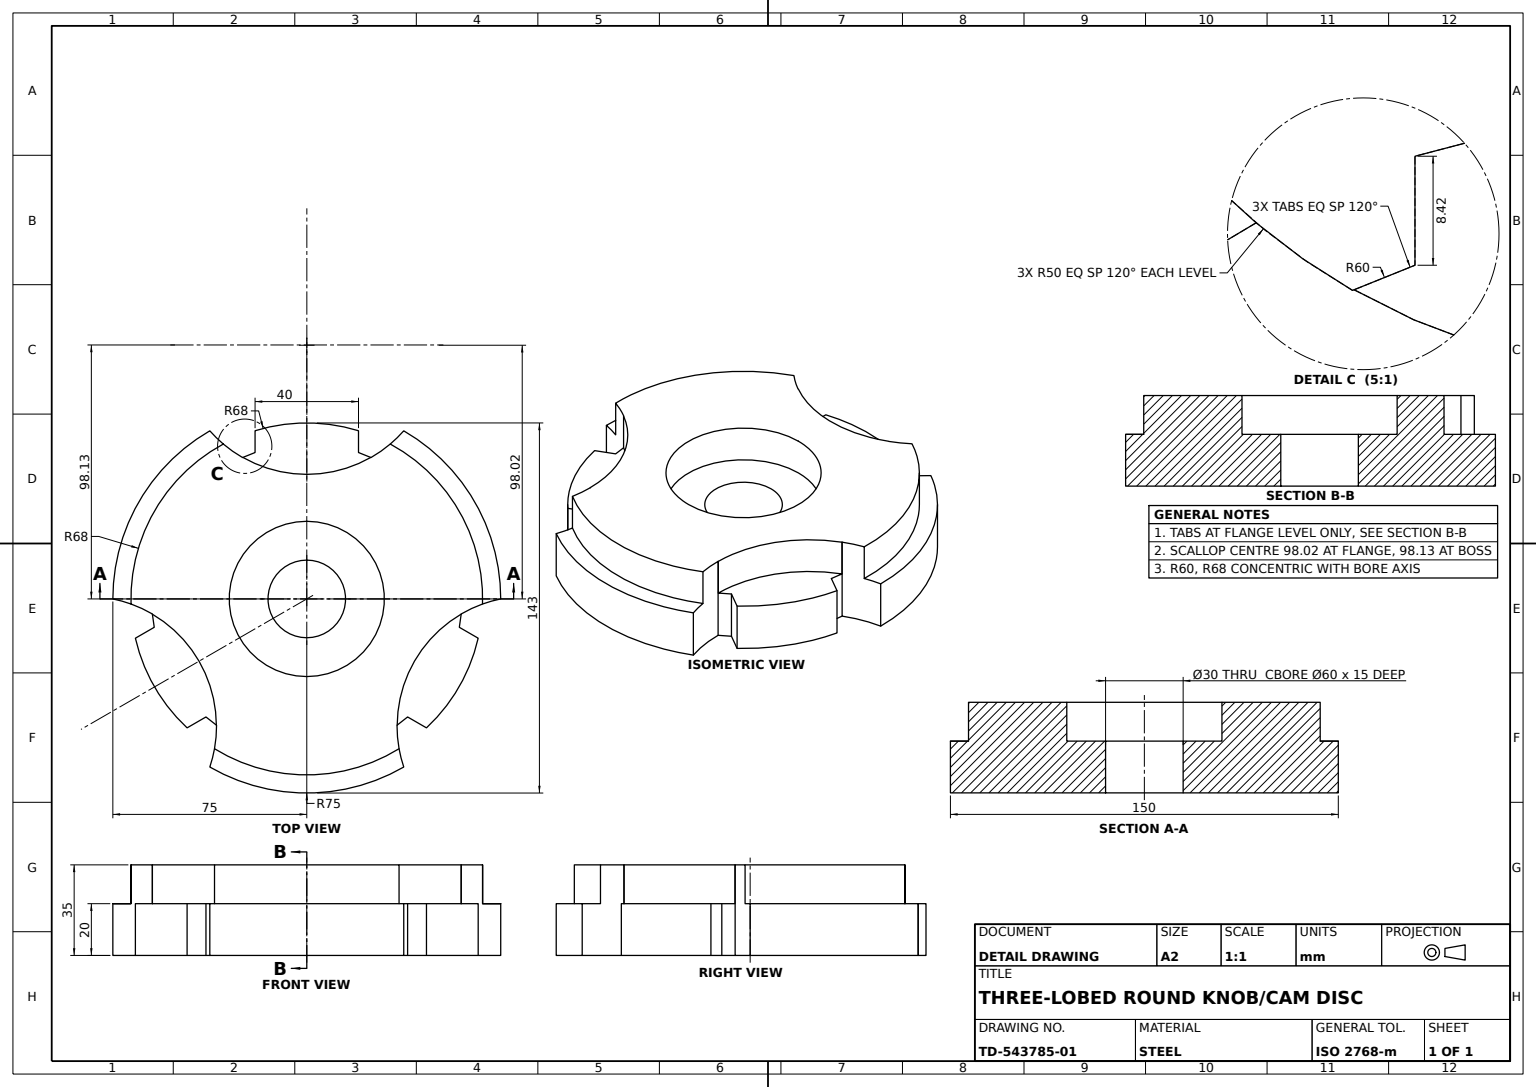
ISO-10303-21;
HEADER;
FILE_DESCRIPTION((''),'2;1');
FILE_NAME('','',(''),(''),'','','');
FILE_SCHEMA(('AUTOMOTIVE_DESIGN'));
ENDSEC;
DATA;
#1=APPLICATION_CONTEXT('');
#2=PRODUCT_CONTEXT('',#1,'mechanical');
#3=PRODUCT('','','',(#2));
#4=PRODUCT_DEFINITION_FORMATION('','',#3);
#5=PRODUCT_DEFINITION_CONTEXT('',#1,'design');
#6=PRODUCT_DEFINITION('','',#4,#5);
#7=PRODUCT_DEFINITION_SHAPE('','',#6);
#8=(LENGTH_UNIT()NAMED_UNIT(*)SI_UNIT(.MILLI.,.METRE.));
#9=(NAMED_UNIT(*)PLANE_ANGLE_UNIT()SI_UNIT($,.RADIAN.));
#10=(NAMED_UNIT(*)SI_UNIT($,.STERADIAN.)SOLID_ANGLE_UNIT());
#11=UNCERTAINTY_MEASURE_WITH_UNIT(LENGTH_MEASURE(1.E-05),#8,'distance_accuracy_value','');
#12=(GEOMETRIC_REPRESENTATION_CONTEXT(3)GLOBAL_UNCERTAINTY_ASSIGNED_CONTEXT((#11))GLOBAL_UNIT_ASSIGNED_CONTEXT((#8,#9,#10))REPRESENTATION_CONTEXT('',''));
#13=CARTESIAN_POINT('',(59.717933,0.,5.811068));
#14=VERTEX_POINT('',#13);
#15=CARTESIAN_POINT('',(59.717933,35.,5.811068));
#16=VERTEX_POINT('',#15);
#17=DIRECTION('',(0.,1.,0.));
#18=VECTOR('',#17,1000.);
#19=LINE('',#13,#18);
#20=EDGE_CURVE('',#14,#16,#19,.T.);
#21=ORIENTED_EDGE('',*,*,#20,.T.);
#22=CARTESIAN_POINT('',(59.713067,35.,5.860857));
#23=VERTEX_POINT('',#22);
#24=CARTESIAN_POINT('',(0.,35.,0.));
#25=DIRECTION('',(0.,0.,1.));
#26=AXIS2_PLACEMENT_3D('',#24,#17,#25);
#27=CIRCLE('',#26,60.);
#28=EDGE_CURVE('',#23,#16,#27,.T.);
#29=ORIENTED_EDGE('',*,*,#28,.F.);
#30=CARTESIAN_POINT('',(59.713067,20.,5.860857));
#31=VERTEX_POINT('',#30);
#32=DIRECTION('',(0.,-1.,0.));
#33=VECTOR('',#32,1000.);
#34=LINE('',#22,#33);
#35=EDGE_CURVE('',#23,#31,#34,.T.);
#36=ORIENTED_EDGE('',*,*,#35,.T.);
#37=CARTESIAN_POINT('',(58.989795,20.,10.963763));
#38=VERTEX_POINT('',#37);
#39=CARTESIAN_POINT('',(0.,20.,0.));
#40=AXIS2_PLACEMENT_3D('',#39,#17,#25);
#41=CIRCLE('',#40,60.);
#42=EDGE_CURVE('',#38,#31,#41,.T.);
#43=ORIENTED_EDGE('',*,*,#42,.F.);
#44=CARTESIAN_POINT('',(58.989795,0.,10.963763));
#45=VERTEX_POINT('',#44);
#46=LINE('',#44,#18);
#47=EDGE_CURVE('',#45,#38,#46,.T.);
#48=ORIENTED_EDGE('',*,*,#47,.F.);
#49=CARTESIAN_POINT('',(0.,0.,0.));
#50=AXIS2_PLACEMENT_3D('',#49,#17,#25);
#51=CIRCLE('',#50,60.);
#52=EDGE_CURVE('',#45,#14,#51,.T.);
#53=ORIENTED_EDGE('',*,*,#52,.T.);
#54=EDGE_LOOP('',(#21,#29,#36,#43,#48,#53));
#55=FACE_OUTER_BOUND('',#54,.T.);
#56=CYLINDRICAL_SURFACE('',#50,60.);
#57=ADVANCED_FACE('',(#55),#56,.T.);
#58=CARTESIAN_POINT('',(-59.717933,35.,5.811068));
#59=VERTEX_POINT('',#58);
#60=CARTESIAN_POINT('',(-59.709065,35.,5.90149));
#61=VERTEX_POINT('',#60);
#62=EDGE_CURVE('',#59,#61,#27,.T.);
#63=ORIENTED_EDGE('',*,*,#62,.F.);
#64=CARTESIAN_POINT('',(-59.717933,0.,5.811068));
#65=VERTEX_POINT('',#64);
#66=LINE('',#64,#18);
#67=EDGE_CURVE('',#65,#59,#66,.T.);
#68=ORIENTED_EDGE('',*,*,#67,.F.);
#69=CARTESIAN_POINT('',(-58.989795,0.,10.963763));
#70=VERTEX_POINT('',#69);
#71=EDGE_CURVE('',#65,#70,#51,.T.);
#72=ORIENTED_EDGE('',*,*,#71,.T.);
#73=CARTESIAN_POINT('',(-58.989795,20.,10.963763));
#74=VERTEX_POINT('',#73);
#75=LINE('',#69,#18);
#76=EDGE_CURVE('',#70,#74,#75,.T.);
#77=ORIENTED_EDGE('',*,*,#76,.T.);
#78=CARTESIAN_POINT('',(-59.709065,20.,5.90149));
#79=VERTEX_POINT('',#78);
#80=EDGE_CURVE('',#79,#74,#41,.T.);
#81=ORIENTED_EDGE('',*,*,#80,.F.);
#82=LINE('',#60,#33);
#83=EDGE_CURVE('',#61,#79,#82,.T.);
#84=ORIENTED_EDGE('',*,*,#83,.F.);
#85=EDGE_LOOP('',(#63,#68,#72,#77,#81,#84));
#86=FACE_OUTER_BOUND('',#85,.T.);
#87=ADVANCED_FACE('',(#86),#56,.T.);
#88=CARTESIAN_POINT('',(0.,35.,30.));
#89=VERTEX_POINT('',#88);
#90=CARTESIAN_POINT('',(0.,35.,-30.));
#91=VERTEX_POINT('',#90);
#92=CIRCLE('',#26,30.);
#93=EDGE_CURVE('',#89,#91,#92,.T.);
#94=ORIENTED_EDGE('',*,*,#93,.T.);
#95=CARTESIAN_POINT('',(0.,20.,-30.));
#96=VERTEX_POINT('',#95);
#97=LINE('',#95,#18);
#98=EDGE_CURVE('',#96,#91,#97,.T.);
#99=ORIENTED_EDGE('',*,*,#98,.F.);
#100=CARTESIAN_POINT('',(0.,20.,30.));
#101=VERTEX_POINT('',#100);
#102=CIRCLE('',#40,30.);
#103=EDGE_CURVE('',#101,#96,#102,.T.);
#104=ORIENTED_EDGE('',*,*,#103,.F.);
#105=LINE('',#100,#18);
#106=EDGE_CURVE('',#101,#89,#105,.T.);
#107=ORIENTED_EDGE('',*,*,#106,.T.);
#108=EDGE_LOOP('',(#94,#99,#104,#107));
#109=FACE_OUTER_BOUND('',#108,.T.);
#110=CYLINDRICAL_SURFACE('',#40,30.);
#111=ADVANCED_FACE('',(#109),#110,.F.);
#112=ORIENTED_EDGE('',*,*,#35,.F.);
#113=CARTESIAN_POINT('',(34.958951,35.,48.763426));
#114=VERTEX_POINT('',#113);
#115=CARTESIAN_POINT('',(84.958295,35.,49.019616));
#116=AXIS2_PLACEMENT_3D('',#115,#17,#25);
#117=CIRCLE('',#116,50.);
#118=EDGE_CURVE('',#23,#114,#117,.T.);
#119=ORIENTED_EDGE('',*,*,#118,.T.);
#120=CARTESIAN_POINT('',(34.958951,20.,48.763426));
#121=VERTEX_POINT('',#120);
#122=LINE('',#113,#33);
#123=EDGE_CURVE('',#114,#121,#122,.T.);
#124=ORIENTED_EDGE('',*,*,#123,.T.);
#125=CARTESIAN_POINT('',(84.958295,20.,49.019616));
#126=AXIS2_PLACEMENT_3D('',#125,#17,#25);
#127=CIRCLE('',#126,50.);
#128=EDGE_CURVE('',#31,#121,#127,.T.);
#129=ORIENTED_EDGE('',*,*,#128,.F.);
#130=EDGE_LOOP('',(#112,#119,#124,#129));
#131=FACE_OUTER_BOUND('',#130,.T.);
#132=DIRECTION('',(0.,0.,-1.));
#133=AXIS2_PLACEMENT_3D('',#115,#32,#132);
#134=CYLINDRICAL_SURFACE('',#133,50.);
#135=ADVANCED_FACE('',(#131),#134,.F.);
#136=CARTESIAN_POINT('',(20.,0.,-64.992307));
#137=VERTEX_POINT('',#136);
#138=CARTESIAN_POINT('',(20.,20.,-64.992307));
#139=VERTEX_POINT('',#138);
#140=LINE('',#136,#18);
#141=EDGE_CURVE('',#137,#139,#140,.T.);
#142=ORIENTED_EDGE('',*,*,#141,.T.);
#143=CARTESIAN_POINT('',(20.,20.,-56.568542));
#144=VERTEX_POINT('',#143);
#145=VECTOR('',#132,1000.);
#146=LINE('',#138,#145);
#147=EDGE_CURVE('',#144,#139,#146,.T.);
#148=ORIENTED_EDGE('',*,*,#147,.F.);
#149=CARTESIAN_POINT('',(20.,0.,-56.568542));
#150=VERTEX_POINT('',#149);
#151=LINE('',#149,#18);
#152=EDGE_CURVE('',#150,#144,#151,.T.);
#153=ORIENTED_EDGE('',*,*,#152,.F.);
#154=LINE('',#136,#145);
#155=EDGE_CURVE('',#150,#137,#154,.T.);
#156=ORIENTED_EDGE('',*,*,#155,.T.);
#157=EDGE_LOOP('',(#142,#148,#153,#156));
#158=FACE_OUTER_BOUND('',#157,.T.);
#159=DIRECTION('',(1.,0.,0.));
#160=AXIS2_PLACEMENT_3D('',#136,#159,#132);
#161=PLANE('',#160);
#162=ADVANCED_FACE('',(#158),#161,.T.);
#163=CARTESIAN_POINT('',(-24.712485,35.,-54.674428));
#164=VERTEX_POINT('',#163);
#165=CARTESIAN_POINT('',(-24.712485,20.,-54.674428));
#166=VERTEX_POINT('',#165);
#167=LINE('',#163,#33);
#168=EDGE_CURVE('',#164,#166,#167,.T.);
#169=ORIENTED_EDGE('',*,*,#168,.F.);
#170=CARTESIAN_POINT('',(24.737649,35.,-54.663047));
#171=VERTEX_POINT('',#170);
#172=CARTESIAN_POINT('',(0.022584,35.,-98.12758));
#173=AXIS2_PLACEMENT_3D('',#172,#17,#25);
#174=CIRCLE('',#173,50.);
#175=EDGE_CURVE('',#164,#171,#174,.T.);
#176=ORIENTED_EDGE('',*,*,#175,.T.);
#177=CARTESIAN_POINT('',(24.737649,20.,-54.663047));
#178=VERTEX_POINT('',#177);
#179=LINE('',#170,#33);
#180=EDGE_CURVE('',#171,#178,#179,.T.);
#181=ORIENTED_EDGE('',*,*,#180,.T.);
#182=CARTESIAN_POINT('',(0.022584,20.,-98.12758));
#183=AXIS2_PLACEMENT_3D('',#182,#17,#25);
#184=CIRCLE('',#183,50.);
#185=EDGE_CURVE('',#166,#178,#184,.T.);
#186=ORIENTED_EDGE('',*,*,#185,.F.);
#187=EDGE_LOOP('',(#169,#176,#181,#186));
#188=FACE_OUTER_BOUND('',#187,.T.);
#189=AXIS2_PLACEMENT_3D('',#172,#32,#132);
#190=CYLINDRICAL_SURFACE('',#189,50.);
#191=ADVANCED_FACE('',(#188),#190,.F.);
#192=CARTESIAN_POINT('',(-24.826434,0.,-54.622781));
#193=VERTEX_POINT('',#192);
#194=CARTESIAN_POINT('',(-37.5,0.,-64.951905));
#195=VERTEX_POINT('',#194);
#196=CARTESIAN_POINT('',(0.,0.,-98.023797));
#197=AXIS2_PLACEMENT_3D('',#196,#32,#132);
#198=CIRCLE('',#197,50.);
#199=EDGE_CURVE('',#193,#195,#198,.T.);
#200=ORIENTED_EDGE('',*,*,#199,.T.);
#201=CARTESIAN_POINT('',(-37.5,20.,-64.951905));
#202=VERTEX_POINT('',#201);
#203=LINE('',#201,#33);
#204=EDGE_CURVE('',#202,#195,#203,.T.);
#205=ORIENTED_EDGE('',*,*,#204,.F.);
#206=CARTESIAN_POINT('',(-32.287087,20.,-59.846002));
#207=VERTEX_POINT('',#206);
#208=CARTESIAN_POINT('',(0.,20.,-98.023797));
#209=AXIS2_PLACEMENT_3D('',#208,#32,#132);
#210=CIRCLE('',#209,50.);
#211=EDGE_CURVE('',#207,#202,#210,.T.);
#212=ORIENTED_EDGE('',*,*,#211,.F.);
#213=CARTESIAN_POINT('',(-32.287087,35.,-59.846002));
#214=VERTEX_POINT('',#213);
#215=LINE('',#213,#33);
#216=EDGE_CURVE('',#214,#207,#215,.T.);
#217=ORIENTED_EDGE('',*,*,#216,.F.);
#218=CARTESIAN_POINT('',(-24.826434,35.,-54.622781));
#219=VERTEX_POINT('',#218);
#220=CARTESIAN_POINT('',(0.,35.,-98.023797));
#221=AXIS2_PLACEMENT_3D('',#220,#32,#25);
#222=CIRCLE('',#221,50.);
#223=EDGE_CURVE('',#219,#214,#222,.T.);
#224=ORIENTED_EDGE('',*,*,#223,.F.);
#225=LINE('',#192,#18);
#226=EDGE_CURVE('',#193,#219,#225,.T.);
#227=ORIENTED_EDGE('',*,*,#226,.F.);
#228=EDGE_LOOP('',(#200,#205,#212,#217,#224,#227));
#229=FACE_OUTER_BOUND('',#228,.T.);
#230=CYLINDRICAL_SURFACE('',#209,50.);
#231=ADVANCED_FACE('',(#229),#230,.F.);
#232=CARTESIAN_POINT('',(-67.971702,20.,1.961563));
#233=VERTEX_POINT('',#232);
#234=CIRCLE('',#40,68.);
#235=EDGE_CURVE('',#207,#233,#234,.T.);
#236=ORIENTED_EDGE('',*,*,#235,.T.);
#237=CARTESIAN_POINT('',(-67.971702,35.,1.961563));
#238=VERTEX_POINT('',#237);
#239=LINE('',#237,#33);
#240=EDGE_CURVE('',#238,#233,#239,.T.);
#241=ORIENTED_EDGE('',*,*,#240,.F.);
#242=CIRCLE('',#26,68.);
#243=EDGE_CURVE('',#214,#238,#242,.T.);
#244=ORIENTED_EDGE('',*,*,#243,.F.);
#245=ORIENTED_EDGE('',*,*,#216,.T.);
#246=EDGE_LOOP('',(#236,#241,#244,#245));
#247=FACE_OUTER_BOUND('',#246,.T.);
#248=AXIS2_PLACEMENT_3D('',#24,#32,#132);
#249=CYLINDRICAL_SURFACE('',#248,68.);
#250=ADVANCED_FACE('',(#247),#249,.T.);
#251=CARTESIAN_POINT('',(-37.5,20.,64.951905));
#252=VERTEX_POINT('',#251);
#253=CARTESIAN_POINT('',(37.5,20.,64.951905));
#254=VERTEX_POINT('',#253);
#255=CIRCLE('',#40,75.);
#256=EDGE_CURVE('',#252,#254,#255,.T.);
#257=ORIENTED_EDGE('',*,*,#256,.T.);
#258=CARTESIAN_POINT('',(35.684615,20.,57.884439));
#259=VERTEX_POINT('',#258);
#260=CARTESIAN_POINT('',(84.891098,20.,49.011898));
#261=AXIS2_PLACEMENT_3D('',#260,#32,#132);
#262=CIRCLE('',#261,50.);
#263=EDGE_CURVE('',#254,#259,#262,.T.);
#264=ORIENTED_EDGE('',*,*,#263,.T.);
#265=CARTESIAN_POINT('',(-35.684615,20.,57.884439));
#266=VERTEX_POINT('',#265);
#267=EDGE_CURVE('',#266,#259,#234,.T.);
#268=ORIENTED_EDGE('',*,*,#267,.F.);
#269=CARTESIAN_POINT('',(-84.891098,20.,49.011898));
#270=AXIS2_PLACEMENT_3D('',#269,#32,#132);
#271=CIRCLE('',#270,50.);
#272=EDGE_CURVE('',#266,#252,#271,.T.);
#273=ORIENTED_EDGE('',*,*,#272,.T.);
#274=EDGE_LOOP('',(#257,#264,#268,#273));
#275=FACE_OUTER_BOUND('',#274,.T.);
#276=CARTESIAN_POINT('',(-42.445549,20.,24.505949));
#277=AXIS2_PLACEMENT_3D('',#276,#32,#132);
#278=PLANE('',#277);
#279=ADVANCED_FACE('',(#275),#278,.F.);
#280=ORIENTED_EDGE('',*,*,#226,.T.);
#281=EDGE_CURVE('',#164,#219,#27,.T.);
#282=ORIENTED_EDGE('',*,*,#281,.F.);
#283=ORIENTED_EDGE('',*,*,#168,.T.);
#284=CARTESIAN_POINT('',(-20.,20.,-56.568542));
#285=VERTEX_POINT('',#284);
#286=EDGE_CURVE('',#285,#166,#41,.T.);
#287=ORIENTED_EDGE('',*,*,#286,.F.);
#288=CARTESIAN_POINT('',(-20.,0.,-56.568542));
#289=VERTEX_POINT('',#288);
#290=LINE('',#288,#18);
#291=EDGE_CURVE('',#289,#285,#290,.T.);
#292=ORIENTED_EDGE('',*,*,#291,.F.);
#293=EDGE_CURVE('',#289,#193,#51,.T.);
#294=ORIENTED_EDGE('',*,*,#293,.T.);
#295=EDGE_LOOP('',(#280,#282,#283,#287,#292,#294));
#296=FACE_OUTER_BOUND('',#295,.T.);
#297=ADVANCED_FACE('',(#296),#56,.T.);
#298=CARTESIAN_POINT('',(46.284989,20.,49.816662));
#299=VERTEX_POINT('',#298);
#300=CARTESIAN_POINT('',(66.284989,20.,15.175646));
#301=VERTEX_POINT('',#300);
#302=EDGE_CURVE('',#299,#301,#234,.T.);
#303=ORIENTED_EDGE('',*,*,#302,.F.);
#304=CARTESIAN_POINT('',(46.284989,0.,49.816662));
#305=VERTEX_POINT('',#304);
#306=LINE('',#304,#18);
#307=EDGE_CURVE('',#305,#299,#306,.T.);
#308=ORIENTED_EDGE('',*,*,#307,.F.);
#309=CARTESIAN_POINT('',(66.284989,0.,15.175646));
#310=VERTEX_POINT('',#309);
#311=CIRCLE('',#50,68.);
#312=EDGE_CURVE('',#305,#310,#311,.T.);
#313=ORIENTED_EDGE('',*,*,#312,.T.);
#314=LINE('',#309,#18);
#315=EDGE_CURVE('',#310,#301,#314,.T.);
#316=ORIENTED_EDGE('',*,*,#315,.T.);
#317=EDGE_LOOP('',(#303,#308,#313,#316));
#318=FACE_OUTER_BOUND('',#317,.T.);
#319=CYLINDRICAL_SURFACE('',#50,68.);
#320=ADVANCED_FACE('',(#318),#319,.T.);
#321=CARTESIAN_POINT('',(0.,0.,-15.));
#322=VERTEX_POINT('',#321);
#323=CARTESIAN_POINT('',(0.,20.,-15.));
#324=VERTEX_POINT('',#323);
#325=CARTESIAN_POINT('',(0.,-40.,-15.));
#326=LINE('',#325,#18);
#327=EDGE_CURVE('',#322,#324,#326,.T.);
#328=ORIENTED_EDGE('',*,*,#327,.T.);
#329=CARTESIAN_POINT('',(0.,20.,15.));
#330=VERTEX_POINT('',#329);
#331=CIRCLE('',#40,15.);
#332=EDGE_CURVE('',#324,#330,#331,.T.);
#333=ORIENTED_EDGE('',*,*,#332,.T.);
#334=CARTESIAN_POINT('',(0.,0.,15.));
#335=VERTEX_POINT('',#334);
#336=CARTESIAN_POINT('',(0.,-40.,15.));
#337=LINE('',#336,#18);
#338=EDGE_CURVE('',#335,#330,#337,.T.);
#339=ORIENTED_EDGE('',*,*,#338,.F.);
#340=AXIS2_PLACEMENT_3D('',#49,#32,#132);
#341=CIRCLE('',#340,15.);
#342=EDGE_CURVE('',#335,#322,#341,.T.);
#343=ORIENTED_EDGE('',*,*,#342,.T.);
#344=EDGE_LOOP('',(#328,#333,#339,#343));
#345=FACE_OUTER_BOUND('',#344,.T.);
#346=CARTESIAN_POINT('',(0.,-40.,0.));
#347=AXIS2_PLACEMENT_3D('',#346,#17,#25);
#348=CYLINDRICAL_SURFACE('',#347,15.);
#349=ADVANCED_FACE('',(#345),#348,.F.);
#350=CARTESIAN_POINT('',(75.,20.,0.));
#351=VERTEX_POINT('',#350);
#352=CARTESIAN_POINT('',(37.5,20.,-64.951905));
#353=VERTEX_POINT('',#352);
#354=EDGE_CURVE('',#351,#353,#255,.T.);
#355=ORIENTED_EDGE('',*,*,#354,.T.);
#356=CARTESIAN_POINT('',(32.287087,20.,-59.846002));
#357=VERTEX_POINT('',#356);
#358=EDGE_CURVE('',#353,#357,#210,.T.);
#359=ORIENTED_EDGE('',*,*,#358,.T.);
#360=CARTESIAN_POINT('',(67.971702,20.,1.961563));
#361=VERTEX_POINT('',#360);
#362=EDGE_CURVE('',#361,#357,#234,.T.);
#363=ORIENTED_EDGE('',*,*,#362,.F.);
#364=EDGE_CURVE('',#361,#351,#262,.T.);
#365=ORIENTED_EDGE('',*,*,#364,.T.);
#366=EDGE_LOOP('',(#355,#359,#363,#365));
#367=FACE_OUTER_BOUND('',#366,.T.);
#368=ADVANCED_FACE('',(#367),#278,.F.);
#369=CARTESIAN_POINT('',(35.684615,35.,57.884439));
#370=VERTEX_POINT('',#369);
#371=LINE('',#369,#33);
#372=EDGE_CURVE('',#370,#259,#371,.T.);
#373=ORIENTED_EDGE('',*,*,#372,.F.);
#374=CARTESIAN_POINT('',(-35.684615,35.,57.884439));
#375=VERTEX_POINT('',#374);
#376=EDGE_CURVE('',#375,#370,#242,.T.);
#377=ORIENTED_EDGE('',*,*,#376,.F.);
#378=LINE('',#374,#33);
#379=EDGE_CURVE('',#375,#266,#378,.T.);
#380=ORIENTED_EDGE('',*,*,#379,.T.);
#381=ORIENTED_EDGE('',*,*,#267,.T.);
#382=EDGE_LOOP('',(#373,#377,#380,#381));
#383=FACE_OUTER_BOUND('',#382,.T.);
#384=ADVANCED_FACE('',(#383),#249,.T.);
#385=ORIENTED_EDGE('',*,*,#364,.F.);
#386=CARTESIAN_POINT('',(67.971702,35.,1.961563));
#387=VERTEX_POINT('',#386);
#388=LINE('',#386,#33);
#389=EDGE_CURVE('',#387,#361,#388,.T.);
#390=ORIENTED_EDGE('',*,*,#389,.F.);
#391=CARTESIAN_POINT('',(84.891098,35.,49.011898));
#392=AXIS2_PLACEMENT_3D('',#391,#32,#25);
#393=CIRCLE('',#392,50.);
#394=EDGE_CURVE('',#16,#387,#393,.T.);
#395=ORIENTED_EDGE('',*,*,#394,.F.);
#396=ORIENTED_EDGE('',*,*,#20,.F.);
#397=CARTESIAN_POINT('',(75.,0.,0.));
#398=VERTEX_POINT('',#397);
#399=CARTESIAN_POINT('',(84.891098,0.,49.011898));
#400=AXIS2_PLACEMENT_3D('',#399,#32,#132);
#401=CIRCLE('',#400,50.);
#402=EDGE_CURVE('',#14,#398,#401,.T.);
#403=ORIENTED_EDGE('',*,*,#402,.T.);
#404=LINE('',#350,#33);
#405=EDGE_CURVE('',#351,#398,#404,.T.);
#406=ORIENTED_EDGE('',*,*,#405,.F.);
#407=EDGE_LOOP('',(#385,#390,#395,#396,#403,#406));
#408=FACE_OUTER_BOUND('',#407,.T.);
#409=CYLINDRICAL_SURFACE('',#261,50.);
#410=ADVANCED_FACE('',(#408),#409,.F.);
#411=CARTESIAN_POINT('',(24.826434,35.,-54.622781));
#412=VERTEX_POINT('',#411);
#413=EDGE_CURVE('',#412,#171,#27,.T.);
#414=ORIENTED_EDGE('',*,*,#413,.F.);
#415=CARTESIAN_POINT('',(24.826434,0.,-54.622781));
#416=VERTEX_POINT('',#415);
#417=LINE('',#415,#18);
#418=EDGE_CURVE('',#416,#412,#417,.T.);
#419=ORIENTED_EDGE('',*,*,#418,.F.);
#420=EDGE_CURVE('',#416,#150,#51,.T.);
#421=ORIENTED_EDGE('',*,*,#420,.T.);
#422=ORIENTED_EDGE('',*,*,#152,.T.);
#423=EDGE_CURVE('',#178,#144,#41,.T.);
#424=ORIENTED_EDGE('',*,*,#423,.F.);
#425=ORIENTED_EDGE('',*,*,#180,.F.);
#426=EDGE_LOOP('',(#414,#419,#421,#422,#424,#425));
#427=FACE_OUTER_BOUND('',#426,.T.);
#428=ADVANCED_FACE('',(#427),#56,.T.);
#429=ORIENTED_EDGE('',*,*,#307,.T.);
#430=CARTESIAN_POINT('',(38.989795,20.,45.604779));
#431=VERTEX_POINT('',#430);
#432=DIRECTION('',(0.866025404,0.,0.5));
#433=VECTOR('',#432,1000.);
#434=LINE('',#298,#433);
#435=EDGE_CURVE('',#431,#299,#434,.T.);
#436=ORIENTED_EDGE('',*,*,#435,.F.);
#437=CARTESIAN_POINT('',(38.989795,0.,45.604779));
#438=VERTEX_POINT('',#437);
#439=LINE('',#437,#18);
#440=EDGE_CURVE('',#438,#431,#439,.T.);
#441=ORIENTED_EDGE('',*,*,#440,.F.);
#442=LINE('',#304,#433);
#443=EDGE_CURVE('',#438,#305,#442,.T.);
#444=ORIENTED_EDGE('',*,*,#443,.T.);
#445=EDGE_LOOP('',(#429,#436,#441,#444));
#446=FACE_OUTER_BOUND('',#445,.T.);
#447=DIRECTION('',(-0.5,0.,0.866025404));
#448=AXIS2_PLACEMENT_3D('',#304,#447,#432);
#449=PLANE('',#448);
#450=ADVANCED_FACE('',(#446),#449,.T.);
#451=ORIENTED_EDGE('',*,*,#342,.F.);
#452=EDGE_CURVE('',#322,#335,#341,.T.);
#453=ORIENTED_EDGE('',*,*,#452,.F.);
#454=EDGE_LOOP('',(#451,#453));
#455=FACE_BOUND('',#454,.T.);
#456=ORIENTED_EDGE('',*,*,#312,.F.);
#457=ORIENTED_EDGE('',*,*,#443,.F.);
#458=CARTESIAN_POINT('',(34.891499,0.,48.811713));
#459=VERTEX_POINT('',#458);
#460=EDGE_CURVE('',#459,#438,#51,.T.);
#461=ORIENTED_EDGE('',*,*,#460,.F.);
#462=CARTESIAN_POINT('',(37.5,0.,64.951905));
#463=VERTEX_POINT('',#462);
#464=EDGE_CURVE('',#463,#459,#401,.T.);
#465=ORIENTED_EDGE('',*,*,#464,.F.);
#466=CARTESIAN_POINT('',(-37.5,0.,64.951905));
#467=VERTEX_POINT('',#466);
#468=CIRCLE('',#50,75.);
#469=EDGE_CURVE('',#467,#463,#468,.T.);
#470=ORIENTED_EDGE('',*,*,#469,.F.);
#471=CARTESIAN_POINT('',(-34.891499,0.,48.811713));
#472=VERTEX_POINT('',#471);
#473=CARTESIAN_POINT('',(-84.891098,0.,49.011898));
#474=AXIS2_PLACEMENT_3D('',#473,#32,#132);
#475=CIRCLE('',#474,50.);
#476=EDGE_CURVE('',#472,#467,#475,.T.);
#477=ORIENTED_EDGE('',*,*,#476,.F.);
#478=CARTESIAN_POINT('',(-38.989795,0.,45.604779));
#479=VERTEX_POINT('',#478);
#480=EDGE_CURVE('',#479,#472,#51,.T.);
#481=ORIENTED_EDGE('',*,*,#480,.F.);
#482=CARTESIAN_POINT('',(-46.284989,0.,49.816662));
#483=VERTEX_POINT('',#482);
#484=DIRECTION('',(0.866025404,0.,-0.5));
#485=VECTOR('',#484,1000.);
#486=LINE('',#482,#485);
#487=EDGE_CURVE('',#483,#479,#486,.T.);
#488=ORIENTED_EDGE('',*,*,#487,.F.);
#489=CARTESIAN_POINT('',(-66.284989,0.,15.175646));
#490=VERTEX_POINT('',#489);
#491=EDGE_CURVE('',#490,#483,#311,.T.);
#492=ORIENTED_EDGE('',*,*,#491,.F.);
#493=DIRECTION('',(-0.866025404,0.,0.5));
#494=VECTOR('',#493,1000.);
#495=LINE('',#489,#494);
#496=EDGE_CURVE('',#70,#490,#495,.T.);
#497=ORIENTED_EDGE('',*,*,#496,.F.);
#498=ORIENTED_EDGE('',*,*,#71,.F.);
#499=CARTESIAN_POINT('',(-75.,0.,0.));
#500=VERTEX_POINT('',#499);
#501=EDGE_CURVE('',#500,#65,#475,.T.);
#502=ORIENTED_EDGE('',*,*,#501,.F.);
#503=EDGE_CURVE('',#195,#500,#468,.T.);
#504=ORIENTED_EDGE('',*,*,#503,.F.);
#505=ORIENTED_EDGE('',*,*,#199,.F.);
#506=ORIENTED_EDGE('',*,*,#293,.F.);
#507=CARTESIAN_POINT('',(-20.,0.,-64.992307));
#508=VERTEX_POINT('',#507);
#509=VECTOR('',#25,1000.);
#510=LINE('',#507,#509);
#511=EDGE_CURVE('',#508,#289,#510,.T.);
#512=ORIENTED_EDGE('',*,*,#511,.F.);
#513=EDGE_CURVE('',#137,#508,#311,.T.);
#514=ORIENTED_EDGE('',*,*,#513,.F.);
#515=ORIENTED_EDGE('',*,*,#155,.F.);
#516=ORIENTED_EDGE('',*,*,#420,.F.);
#517=CARTESIAN_POINT('',(37.5,0.,-64.951905));
#518=VERTEX_POINT('',#517);
#519=EDGE_CURVE('',#518,#416,#198,.T.);
#520=ORIENTED_EDGE('',*,*,#519,.F.);
#521=EDGE_CURVE('',#398,#518,#468,.T.);
#522=ORIENTED_EDGE('',*,*,#521,.F.);
#523=ORIENTED_EDGE('',*,*,#402,.F.);
#524=ORIENTED_EDGE('',*,*,#52,.F.);
#525=DIRECTION('',(-0.866025404,0.,-0.5));
#526=VECTOR('',#525,1000.);
#527=LINE('',#309,#526);
#528=EDGE_CURVE('',#310,#45,#527,.T.);
#529=ORIENTED_EDGE('',*,*,#528,.F.);
#530=EDGE_LOOP('',(#456,#457,#461,#465,#470,#477,#481,#488,#492,#497,#498,#502,#504,#505,#506,#512,#514,#515,#516,#520,#522,#523,#524,#529));
#531=FACE_OUTER_BOUND('',#530,.T.);
#532=CARTESIAN_POINT('',(-42.445549,0.,24.505949));
#533=AXIS2_PLACEMENT_3D('',#532,#32,#132);
#534=PLANE('',#533);
#535=ADVANCED_FACE('',(#455,#531),#534,.T.);
#536=EDGE_CURVE('',#96,#101,#102,.T.);
#537=ORIENTED_EDGE('',*,*,#536,.T.);
#538=ORIENTED_EDGE('',*,*,#103,.T.);
#539=EDGE_LOOP('',(#537,#538));
#540=FACE_OUTER_BOUND('',#539,.T.);
#541=EDGE_CURVE('',#330,#324,#331,.T.);
#542=ORIENTED_EDGE('',*,*,#541,.F.);
#543=ORIENTED_EDGE('',*,*,#332,.F.);
#544=EDGE_LOOP('',(#542,#543));
#545=FACE_BOUND('',#544,.T.);
#546=PLANE('',#40);
#547=ADVANCED_FACE('',(#540,#545),#546,.T.);
#548=LINE('',#251,#33);
#549=EDGE_CURVE('',#252,#467,#548,.T.);
#550=ORIENTED_EDGE('',*,*,#549,.T.);
#551=ORIENTED_EDGE('',*,*,#469,.T.);
#552=LINE('',#253,#33);
#553=EDGE_CURVE('',#254,#463,#552,.T.);
#554=ORIENTED_EDGE('',*,*,#553,.F.);
#555=ORIENTED_EDGE('',*,*,#256,.F.);
#556=EDGE_LOOP('',(#550,#551,#554,#555));
#557=FACE_OUTER_BOUND('',#556,.T.);
#558=AXIS2_PLACEMENT_3D('',#39,#32,#132);
#559=CYLINDRICAL_SURFACE('',#558,75.);
#560=ADVANCED_FACE('',(#557),#559,.T.);
#561=CARTESIAN_POINT('',(-20.,20.,-64.992307));
#562=VERTEX_POINT('',#561);
#563=LINE('',#507,#18);
#564=EDGE_CURVE('',#508,#562,#563,.T.);
#565=ORIENTED_EDGE('',*,*,#564,.T.);
#566=EDGE_CURVE('',#139,#562,#234,.T.);
#567=ORIENTED_EDGE('',*,*,#566,.F.);
#568=ORIENTED_EDGE('',*,*,#141,.F.);
#569=ORIENTED_EDGE('',*,*,#513,.T.);
#570=EDGE_LOOP('',(#565,#567,#568,#569));
#571=FACE_OUTER_BOUND('',#570,.T.);
#572=ADVANCED_FACE('',(#571),#319,.T.);
#573=ORIENTED_EDGE('',*,*,#93,.F.);
#574=EDGE_CURVE('',#91,#89,#92,.T.);
#575=ORIENTED_EDGE('',*,*,#574,.F.);
#576=EDGE_LOOP('',(#573,#575));
#577=FACE_BOUND('',#576,.T.);
#578=CARTESIAN_POINT('',(-84.891098,35.,49.011898));
#579=AXIS2_PLACEMENT_3D('',#578,#32,#25);
#580=CIRCLE('',#579,50.);
#581=EDGE_CURVE('',#238,#59,#580,.T.);
#582=ORIENTED_EDGE('',*,*,#581,.T.);
#583=ORIENTED_EDGE('',*,*,#62,.T.);
#584=CARTESIAN_POINT('',(-34.965373,35.,48.758822));
#585=VERTEX_POINT('',#584);
#586=CARTESIAN_POINT('',(-84.9645,35.,49.054277));
#587=AXIS2_PLACEMENT_3D('',#586,#32,#25);
#588=CIRCLE('',#587,50.);
#589=EDGE_CURVE('',#61,#585,#588,.T.);
#590=ORIENTED_EDGE('',*,*,#589,.T.);
#591=CARTESIAN_POINT('',(-34.891499,35.,48.811713));
#592=VERTEX_POINT('',#591);
#593=EDGE_CURVE('',#585,#592,#27,.T.);
#594=ORIENTED_EDGE('',*,*,#593,.T.);
#595=EDGE_CURVE('',#592,#375,#580,.T.);
#596=ORIENTED_EDGE('',*,*,#595,.T.);
#597=ORIENTED_EDGE('',*,*,#376,.T.);
#598=CARTESIAN_POINT('',(34.891499,35.,48.811713));
#599=VERTEX_POINT('',#598);
#600=EDGE_CURVE('',#370,#599,#393,.T.);
#601=ORIENTED_EDGE('',*,*,#600,.T.);
#602=EDGE_CURVE('',#599,#114,#27,.T.);
#603=ORIENTED_EDGE('',*,*,#602,.T.);
#604=ORIENTED_EDGE('',*,*,#118,.F.);
#605=ORIENTED_EDGE('',*,*,#28,.T.);
#606=ORIENTED_EDGE('',*,*,#394,.T.);
#607=CARTESIAN_POINT('',(32.287087,35.,-59.846002));
#608=VERTEX_POINT('',#607);
#609=EDGE_CURVE('',#387,#608,#242,.T.);
#610=ORIENTED_EDGE('',*,*,#609,.T.);
#611=EDGE_CURVE('',#608,#412,#222,.T.);
#612=ORIENTED_EDGE('',*,*,#611,.T.);
#613=ORIENTED_EDGE('',*,*,#413,.T.);
#614=ORIENTED_EDGE('',*,*,#175,.F.);
#615=ORIENTED_EDGE('',*,*,#281,.T.);
#616=ORIENTED_EDGE('',*,*,#223,.T.);
#617=ORIENTED_EDGE('',*,*,#243,.T.);
#618=EDGE_LOOP('',(#582,#583,#590,#594,#596,#597,#601,#603,#604,#605,#606,#610,#612,#613,#614,#615,#616,#617));
#619=FACE_OUTER_BOUND('',#618,.T.);
#620=PLANE('',#26);
#621=ADVANCED_FACE('',(#577,#619),#620,.T.);
#622=ORIENTED_EDGE('',*,*,#487,.T.);
#623=CARTESIAN_POINT('',(-38.989795,20.,45.604779));
#624=VERTEX_POINT('',#623);
#625=LINE('',#478,#18);
#626=EDGE_CURVE('',#479,#624,#625,.T.);
#627=ORIENTED_EDGE('',*,*,#626,.T.);
#628=CARTESIAN_POINT('',(-46.284989,20.,49.816662));
#629=VERTEX_POINT('',#628);
#630=LINE('',#628,#485);
#631=EDGE_CURVE('',#629,#624,#630,.T.);
#632=ORIENTED_EDGE('',*,*,#631,.F.);
#633=LINE('',#482,#18);
#634=EDGE_CURVE('',#483,#629,#633,.T.);
#635=ORIENTED_EDGE('',*,*,#634,.F.);
#636=EDGE_LOOP('',(#622,#627,#632,#635));
#637=FACE_OUTER_BOUND('',#636,.T.);
#638=DIRECTION('',(0.5,0.,0.866025404));
#639=AXIS2_PLACEMENT_3D('',#482,#638,#484);
#640=PLANE('',#639);
#641=ADVANCED_FACE('',(#637),#640,.T.);
#642=ORIENTED_EDGE('',*,*,#564,.F.);
#643=ORIENTED_EDGE('',*,*,#511,.T.);
#644=ORIENTED_EDGE('',*,*,#291,.T.);
#645=LINE('',#561,#509);
#646=EDGE_CURVE('',#562,#285,#645,.T.);
#647=ORIENTED_EDGE('',*,*,#646,.F.);
#648=EDGE_LOOP('',(#642,#643,#644,#647));
#649=FACE_OUTER_BOUND('',#648,.T.);
#650=DIRECTION('',(-1.,0.,0.));
#651=AXIS2_PLACEMENT_3D('',#507,#650,#25);
#652=PLANE('',#651);
#653=ADVANCED_FACE('',(#649),#652,.T.);
#654=ORIENTED_EDGE('',*,*,#611,.F.);
#655=LINE('',#607,#33);
#656=EDGE_CURVE('',#608,#357,#655,.T.);
#657=ORIENTED_EDGE('',*,*,#656,.T.);
#658=ORIENTED_EDGE('',*,*,#358,.F.);
#659=LINE('',#352,#33);
#660=EDGE_CURVE('',#353,#518,#659,.T.);
#661=ORIENTED_EDGE('',*,*,#660,.T.);
#662=ORIENTED_EDGE('',*,*,#519,.T.);
#663=ORIENTED_EDGE('',*,*,#418,.T.);
#664=EDGE_LOOP('',(#654,#657,#658,#661,#662,#663));
#665=FACE_OUTER_BOUND('',#664,.T.);
#666=ADVANCED_FACE('',(#665),#230,.F.);
#667=CARTESIAN_POINT('',(-75.,20.,0.));
#668=VERTEX_POINT('',#667);
#669=LINE('',#667,#33);
#670=EDGE_CURVE('',#668,#500,#669,.T.);
#671=ORIENTED_EDGE('',*,*,#670,.F.);
#672=EDGE_CURVE('',#202,#668,#255,.T.);
#673=ORIENTED_EDGE('',*,*,#672,.F.);
#674=ORIENTED_EDGE('',*,*,#204,.T.);
#675=ORIENTED_EDGE('',*,*,#503,.T.);
#676=EDGE_LOOP('',(#671,#673,#674,#675));
#677=FACE_OUTER_BOUND('',#676,.T.);
#678=ADVANCED_FACE('',(#677),#559,.T.);
#679=ORIENTED_EDGE('',*,*,#185,.T.);
#680=ORIENTED_EDGE('',*,*,#423,.T.);
#681=ORIENTED_EDGE('',*,*,#147,.T.);
#682=ORIENTED_EDGE('',*,*,#566,.T.);
#683=ORIENTED_EDGE('',*,*,#646,.T.);
#684=ORIENTED_EDGE('',*,*,#286,.T.);
#685=EDGE_LOOP('',(#679,#680,#681,#682,#683,#684));
#686=FACE_OUTER_BOUND('',#685,.T.);
#687=ADVANCED_FACE('',(#686),#278,.F.);
#688=ORIENTED_EDGE('',*,*,#549,.F.);
#689=ORIENTED_EDGE('',*,*,#272,.F.);
#690=ORIENTED_EDGE('',*,*,#379,.F.);
#691=ORIENTED_EDGE('',*,*,#595,.F.);
#692=LINE('',#471,#18);
#693=EDGE_CURVE('',#472,#592,#692,.T.);
#694=ORIENTED_EDGE('',*,*,#693,.F.);
#695=ORIENTED_EDGE('',*,*,#476,.T.);
#696=EDGE_LOOP('',(#688,#689,#690,#691,#694,#695));
#697=FACE_OUTER_BOUND('',#696,.T.);
#698=CYLINDRICAL_SURFACE('',#270,50.);
#699=ADVANCED_FACE('',(#697),#698,.F.);
#700=ORIENTED_EDGE('',*,*,#574,.T.);
#701=ORIENTED_EDGE('',*,*,#106,.F.);
#702=ORIENTED_EDGE('',*,*,#536,.F.);
#703=ORIENTED_EDGE('',*,*,#98,.T.);
#704=EDGE_LOOP('',(#700,#701,#702,#703));
#705=FACE_OUTER_BOUND('',#704,.T.);
#706=ADVANCED_FACE('',(#705),#110,.F.);
#707=LINE('',#300,#526);
#708=EDGE_CURVE('',#301,#38,#707,.T.);
#709=ORIENTED_EDGE('',*,*,#708,.F.);
#710=ORIENTED_EDGE('',*,*,#315,.F.);
#711=ORIENTED_EDGE('',*,*,#528,.T.);
#712=ORIENTED_EDGE('',*,*,#47,.T.);
#713=EDGE_LOOP('',(#709,#710,#711,#712));
#714=FACE_OUTER_BOUND('',#713,.T.);
#715=DIRECTION('',(0.5,0.,-0.866025404));
#716=AXIS2_PLACEMENT_3D('',#309,#715,#525);
#717=PLANE('',#716);
#718=ADVANCED_FACE('',(#714),#717,.T.);
#719=ORIENTED_EDGE('',*,*,#338,.T.);
#720=ORIENTED_EDGE('',*,*,#541,.T.);
#721=ORIENTED_EDGE('',*,*,#327,.F.);
#722=ORIENTED_EDGE('',*,*,#452,.T.);
#723=EDGE_LOOP('',(#719,#720,#721,#722));
#724=FACE_OUTER_BOUND('',#723,.T.);
#725=ADVANCED_FACE('',(#724),#348,.F.);
#726=ORIENTED_EDGE('',*,*,#263,.F.);
#727=ORIENTED_EDGE('',*,*,#553,.T.);
#728=ORIENTED_EDGE('',*,*,#464,.T.);
#729=LINE('',#458,#18);
#730=EDGE_CURVE('',#459,#599,#729,.T.);
#731=ORIENTED_EDGE('',*,*,#730,.T.);
#732=ORIENTED_EDGE('',*,*,#600,.F.);
#733=ORIENTED_EDGE('',*,*,#372,.T.);
#734=EDGE_LOOP('',(#726,#727,#728,#731,#732,#733));
#735=FACE_OUTER_BOUND('',#734,.T.);
#736=ADVANCED_FACE('',(#735),#409,.F.);
#737=ORIENTED_EDGE('',*,*,#631,.T.);
#738=CARTESIAN_POINT('',(-34.965373,20.,48.758822));
#739=VERTEX_POINT('',#738);
#740=EDGE_CURVE('',#624,#739,#41,.T.);
#741=ORIENTED_EDGE('',*,*,#740,.T.);
#742=CARTESIAN_POINT('',(-84.9645,20.,49.054277));
#743=AXIS2_PLACEMENT_3D('',#742,#32,#25);
#744=CIRCLE('',#743,50.);
#745=EDGE_CURVE('',#79,#739,#744,.T.);
#746=ORIENTED_EDGE('',*,*,#745,.F.);
#747=ORIENTED_EDGE('',*,*,#80,.T.);
#748=CARTESIAN_POINT('',(-66.284989,20.,15.175646));
#749=VERTEX_POINT('',#748);
#750=LINE('',#748,#494);
#751=EDGE_CURVE('',#74,#749,#750,.T.);
#752=ORIENTED_EDGE('',*,*,#751,.T.);
#753=EDGE_CURVE('',#749,#629,#234,.T.);
#754=ORIENTED_EDGE('',*,*,#753,.T.);
#755=EDGE_LOOP('',(#737,#741,#746,#747,#752,#754));
#756=FACE_OUTER_BOUND('',#755,.T.);
#757=ADVANCED_FACE('',(#756),#278,.F.);
#758=ORIENTED_EDGE('',*,*,#83,.T.);
#759=ORIENTED_EDGE('',*,*,#745,.T.);
#760=LINE('',#584,#33);
#761=EDGE_CURVE('',#585,#739,#760,.T.);
#762=ORIENTED_EDGE('',*,*,#761,.F.);
#763=ORIENTED_EDGE('',*,*,#589,.F.);
#764=EDGE_LOOP('',(#758,#759,#762,#763));
#765=FACE_OUTER_BOUND('',#764,.T.);
#766=AXIS2_PLACEMENT_3D('',#586,#32,#132);
#767=CYLINDRICAL_SURFACE('',#766,50.);
#768=ADVANCED_FACE('',(#765),#767,.F.);
#769=ORIENTED_EDGE('',*,*,#609,.F.);
#770=ORIENTED_EDGE('',*,*,#389,.T.);
#771=ORIENTED_EDGE('',*,*,#362,.T.);
#772=ORIENTED_EDGE('',*,*,#656,.F.);
#773=EDGE_LOOP('',(#769,#770,#771,#772));
#774=FACE_OUTER_BOUND('',#773,.T.);
#775=ADVANCED_FACE('',(#774),#249,.T.);
#776=ORIENTED_EDGE('',*,*,#123,.F.);
#777=ORIENTED_EDGE('',*,*,#602,.F.);
#778=ORIENTED_EDGE('',*,*,#730,.F.);
#779=ORIENTED_EDGE('',*,*,#460,.T.);
#780=ORIENTED_EDGE('',*,*,#440,.T.);
#781=EDGE_CURVE('',#121,#431,#41,.T.);
#782=ORIENTED_EDGE('',*,*,#781,.F.);
#783=EDGE_LOOP('',(#776,#777,#778,#779,#780,#782));
#784=FACE_OUTER_BOUND('',#783,.T.);
#785=ADVANCED_FACE('',(#784),#56,.T.);
#786=ORIENTED_EDGE('',*,*,#42,.T.);
#787=ORIENTED_EDGE('',*,*,#128,.T.);
#788=ORIENTED_EDGE('',*,*,#781,.T.);
#789=ORIENTED_EDGE('',*,*,#435,.T.);
#790=ORIENTED_EDGE('',*,*,#302,.T.);
#791=ORIENTED_EDGE('',*,*,#708,.T.);
#792=EDGE_LOOP('',(#786,#787,#788,#789,#790,#791));
#793=FACE_OUTER_BOUND('',#792,.T.);
#794=ADVANCED_FACE('',(#793),#278,.F.);
#795=ORIENTED_EDGE('',*,*,#521,.T.);
#796=ORIENTED_EDGE('',*,*,#660,.F.);
#797=ORIENTED_EDGE('',*,*,#354,.F.);
#798=ORIENTED_EDGE('',*,*,#405,.T.);
#799=EDGE_LOOP('',(#795,#796,#797,#798));
#800=FACE_OUTER_BOUND('',#799,.T.);
#801=ADVANCED_FACE('',(#800),#559,.T.);
#802=ORIENTED_EDGE('',*,*,#753,.F.);
#803=LINE('',#489,#18);
#804=EDGE_CURVE('',#490,#749,#803,.T.);
#805=ORIENTED_EDGE('',*,*,#804,.F.);
#806=ORIENTED_EDGE('',*,*,#491,.T.);
#807=ORIENTED_EDGE('',*,*,#634,.T.);
#808=EDGE_LOOP('',(#802,#805,#806,#807));
#809=FACE_OUTER_BOUND('',#808,.T.);
#810=ADVANCED_FACE('',(#809),#319,.T.);
#811=ORIENTED_EDGE('',*,*,#693,.T.);
#812=ORIENTED_EDGE('',*,*,#593,.F.);
#813=ORIENTED_EDGE('',*,*,#761,.T.);
#814=ORIENTED_EDGE('',*,*,#740,.F.);
#815=ORIENTED_EDGE('',*,*,#626,.F.);
#816=ORIENTED_EDGE('',*,*,#480,.T.);
#817=EDGE_LOOP('',(#811,#812,#813,#814,#815,#816));
#818=FACE_OUTER_BOUND('',#817,.T.);
#819=ADVANCED_FACE('',(#818),#56,.T.);
#820=ORIENTED_EDGE('',*,*,#804,.T.);
#821=ORIENTED_EDGE('',*,*,#751,.F.);
#822=ORIENTED_EDGE('',*,*,#76,.F.);
#823=ORIENTED_EDGE('',*,*,#496,.T.);
#824=EDGE_LOOP('',(#820,#821,#822,#823));
#825=FACE_OUTER_BOUND('',#824,.T.);
#826=DIRECTION('',(-0.5,0.,-0.866025404));
#827=AXIS2_PLACEMENT_3D('',#489,#826,#493);
#828=PLANE('',#827);
#829=ADVANCED_FACE('',(#825),#828,.T.);
#830=EDGE_CURVE('',#668,#233,#271,.T.);
#831=ORIENTED_EDGE('',*,*,#830,.T.);
#832=ORIENTED_EDGE('',*,*,#235,.F.);
#833=ORIENTED_EDGE('',*,*,#211,.T.);
#834=ORIENTED_EDGE('',*,*,#672,.T.);
#835=EDGE_LOOP('',(#831,#832,#833,#834));
#836=FACE_OUTER_BOUND('',#835,.T.);
#837=ADVANCED_FACE('',(#836),#278,.F.);
#838=ORIENTED_EDGE('',*,*,#670,.T.);
#839=ORIENTED_EDGE('',*,*,#501,.T.);
#840=ORIENTED_EDGE('',*,*,#67,.T.);
#841=ORIENTED_EDGE('',*,*,#581,.F.);
#842=ORIENTED_EDGE('',*,*,#240,.T.);
#843=ORIENTED_EDGE('',*,*,#830,.F.);
#844=EDGE_LOOP('',(#838,#839,#840,#841,#842,#843));
#845=FACE_OUTER_BOUND('',#844,.T.);
#846=ADVANCED_FACE('',(#845),#698,.F.);
#847=CLOSED_SHELL('',(#57,#87,#111,#135,#162,#191,#231,#250,#279,#297,#320,#349,#368,#384,#410,#428,#450,#535,#547,#560,#572,#621,#641,#653,#666,#678,#687,#699,#706,#718,#725,#736,#757,#768,#775,#785,#794,#801,#810,#819,#829,#837,#846));
#848=MANIFOLD_SOLID_BREP('',#847);
#849=ADVANCED_BREP_SHAPE_REPRESENTATION('',(#848),#12);
#850=SHAPE_DEFINITION_REPRESENTATION(#7,#849);
ENDSEC;
END-ISO-10303-21;
